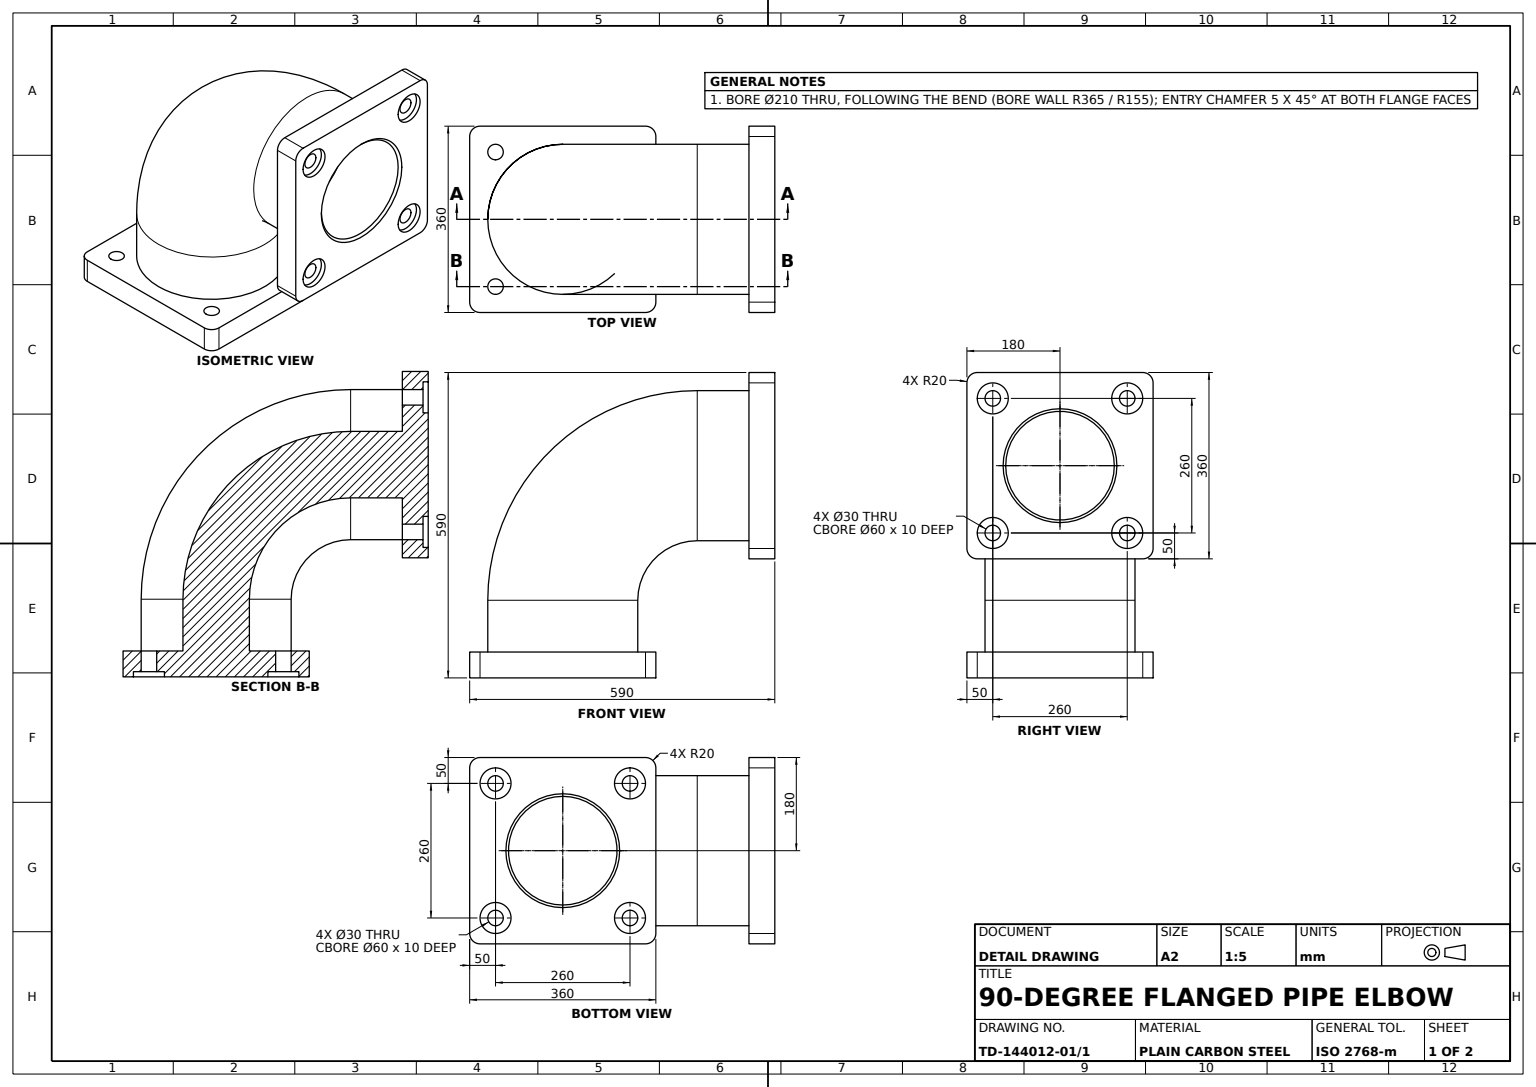
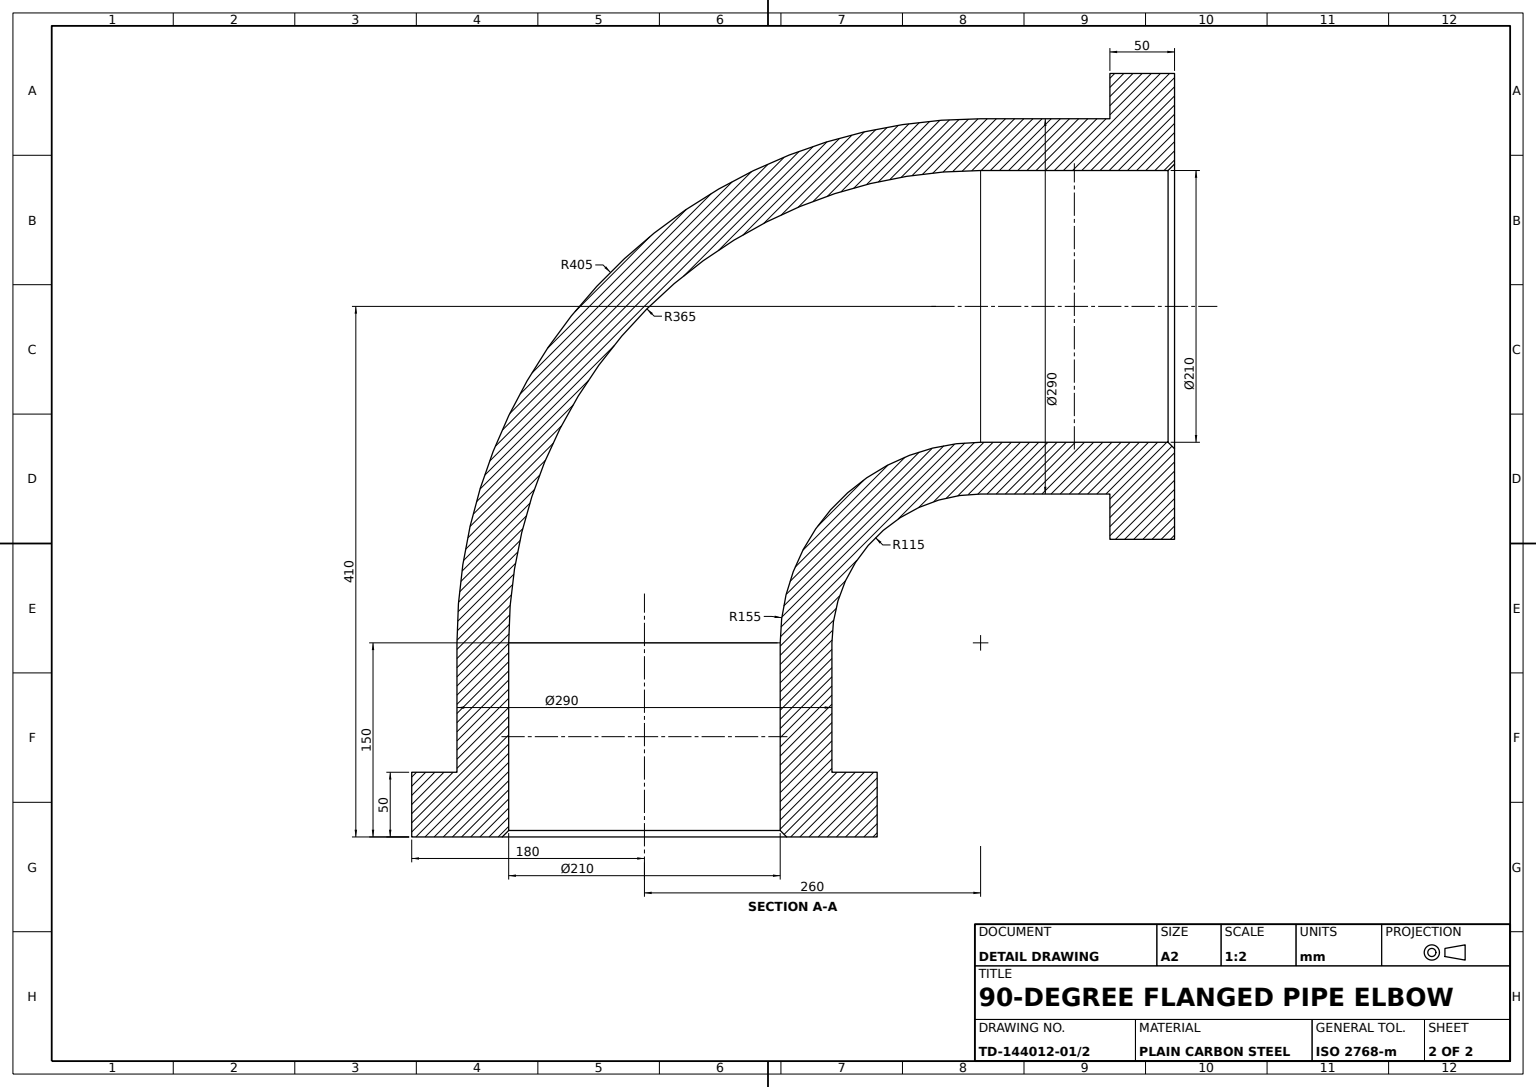
solid
v1 (-130,50,115)
v2 (-130,10,115)
e1 v1 v2 LINE
v3 (-130,50,145)
e2 v3 v1 CIRCLE(AX(P(-130,50,130),D(0,-1,0),D(0,0,-1)),15)
v4 (-130,10,145)
e3 v3 v4 LINE
e4 v2 v4 CIRCLE(AX(P(-130,10,130),D(0,1,0),D(0,0,-1)),15)
face CYL(AX(P(-130,50,130),D(0,-1,0),D(0,0,-1)),15) rev [-e1 -e2 e3 -e4]
v5 (-130,10,100)
v6 (-130,10,160)
e5 v5 v6 CIRCLE(AX(P(-130,10,130),D(0,-1,0),D(0,0,-1)),30)
e6 v6 v5 CIRCLE(AX(P(-130,10,130),D(0,-1,0),D(0,0,-1)),30)
e7 v4 v2 CIRCLE(AX(P(-130,10,130),D(0,1,0),D(0,0,-1)),15)
face PLANE(AX(P(-130,10,130),D(0,-1,0),D(0,0,-1))) [e5 e6] [e7 e4]
v7 (360,540,115)
v8 (400,540,115)
e8 v7 v8 LINE
v9 (400,540,145)
e9 v9 v8 CIRCLE(AX(P(400,540,130),D(-1,0,0),D(0,0,-1)),15)
v10 (360,540,145)
e10 v10 v9 LINE
e11 v7 v10 CIRCLE(AX(P(360,540,130),D(1,0,0),D(0,0,-1)),15)
face CYL(AX(P(360,540,130),D(1,0,0),D(0,0,-1)),15) rev [e8 -e9 -e10 -e11]
v11 (0,0,-110)
v12 (0,0,110)
e12 v11 v12 CIRCLE(AX(P(0,0,0),D(0,1,0),D(0,0,1)),110)
v13 (0,5,-105)
e13 v13 v11 LINE
v14 (0,5,105)
e14 v14 v13 CIRCLE(AX(P(0,5,0),D(0,-1,0),D(0,0,1)),105)
e15 v14 v12 LINE
face CONE(AX(P(0,5,0),D(0,-1,0),D(0,0,-1)),105,0.785398163) rev [-e12 -e13 -e14 e15]
v15 (410,540,160)
v16 (410,540,100)
e16 v15 v16 CIRCLE(AX(P(410,540,130),D(1,0,0),D(0,0,-1)),30)
v17 (400,540,100)
e17 v17 v16 LINE
v18 (400,540,160)
e18 v18 v17 CIRCLE(AX(P(400,540,130),D(1,0,0),D(0,0,-1)),30)
e19 v18 v15 LINE
face CYL(AX(P(400,540,130),D(1,0,0),D(0,0,-1)),30) rev [e16 -e17 -e18 e19]
v19 (0,150,-105)
v20 (105,150,0)
e20 v19 v20 CIRCLE(AX(P(0,150,0),D(0,-1,0),D(0,0,-1)),105)
e21 v13 v19 LINE
e22 v13 v14 CIRCLE(AX(P(0,5,0),D(0,-1,0),D(0,0,1)),105)
v21 (0,150,105)
e23 v14 v21 LINE
e24 v20 v21 CIRCLE(AX(P(0,150,0),D(0,-1,0),D(0,0,-1)),105)
face CYL(AX(P(0,0,0),D(0,1,0),D(0,0,1)),105) rev [-e20 -e21 e22 e23 -e24]
e25 v1 v3 CIRCLE(AX(P(-130,50,130),D(0,-1,0),D(0,0,-1)),15)
face CYL(AX(P(-130,50,130),D(0,-1,0),D(0,0,-1)),15) rev [-e25 e1 -e7 -e3]
v22 (360,280,-115)
v23 (360,280,-145)
e26 v22 v23 CIRCLE(AX(P(360,280,-130),D(1,0,0),D(0,0,1)),15)
v24 (400,280,-115)
e27 v22 v24 LINE
v25 (400,280,-145)
e28 v25 v24 CIRCLE(AX(P(400,280,-130),D(-1,0,0),D(0,0,-1)),15)
e29 v23 v25 LINE
face CYL(AX(P(360,280,-130),D(1,0,0),D(0,0,-1)),15) rev [-e26 e27 -e28 -e29]
v26 (-130,50,-145)
v27 (-130,10,-145)
e30 v26 v27 LINE
v28 (-130,10,-115)
e31 v28 v27 CIRCLE(AX(P(-130,10,-130),D(0,1,0),D(0,0,-1)),15)
v29 (-130,50,-115)
e32 v29 v28 LINE
e33 v26 v29 CIRCLE(AX(P(-130,50,-130),D(0,-1,0),D(0,0,-1)),15)
face CYL(AX(P(-130,50,-130),D(0,-1,0),D(0,0,-1)),15) rev [e30 -e31 -e32 -e33]
v30 (-105,150,0)
e34 v30 v19 CIRCLE(AX(P(0,150,0),D(0,-1,0),D(0,0,-1)),105)
v31 (260,305,0)
e35 v20 v31 CIRCLE(AX(P(260,150,0),D(0,0,-1),D(-1,0,0)),155)
v32 (260,410,-105)
e36 v32 v31 CIRCLE(AX(P(260,410,0),D(-1,0,0),D(0,0,-1)),105)
v33 (260,515,0)
e37 v33 v32 CIRCLE(AX(P(260,410,0),D(-1,0,0),D(0,0,-1)),105)
e38 v30 v33 CIRCLE(AX(P(260,150,0),D(0,0,-1),D(-1,0,0)),365)
face TORUS(AX(P(260,150,0),D(0,0,-1),D(-1,0,0)),260,105) rev [e34 e20 e35 -e36 -e37 -e38]
v34 (400,540,-145)
v35 (400,540,-115)
e39 v34 v35 CIRCLE(AX(P(400,540,-130),D(-1,0,0),D(0,0,-1)),15)
e40 v35 v34 CIRCLE(AX(P(400,540,-130),D(-1,0,0),D(0,0,-1)),15)
v36 (400,540,-100)
v37 (400,540,-160)
e41 v36 v37 CIRCLE(AX(P(400,540,-130),D(1,0,0),D(0,0,-1)),30)
e42 v37 v36 CIRCLE(AX(P(400,540,-130),D(1,0,0),D(0,0,-1)),30)
face PLANE(AX(P(400,540,-130),D(1,0,0),D(0,0,-1))) [e39 e40] [e41 e42]
v38 (360,590,-160)
v39 (360,590,160)
e43 v38 v39 LINE
v40 (410,590,160)
e44 v39 v40 LINE
v41 (410,590,-160)
e45 v41 v40 LINE
e46 v38 v41 LINE
face PLANE(AX(P(360,590,160),D(0,1,0),D(0,0,1))) [e43 e44 -e45 -e46]
v42 (360,570,-180)
v43 (410,570,-180)
e47 v42 v43 LINE
v44 (410,250,-180)
e48 v44 v43 LINE
v45 (360,250,-180)
e49 v45 v44 LINE
e50 v45 v42 LINE
face PLANE(AX(P(360,250,-180),D(0,0,-1),D(-1,0,0))) [e47 -e48 -e49 e50]
v46 (-130,0,100)
v47 (-130,0,160)
e51 v46 v47 CIRCLE(AX(P(-130,0,130),D(0,-1,0),D(0,0,-1)),30)
e52 v6 v47 LINE
e53 v5 v46 LINE
face CYL(AX(P(-130,10,130),D(0,-1,0),D(0,0,-1)),30) rev [e51 -e52 -e5 e53]
e54 v21 v30 CIRCLE(AX(P(0,150,0),D(0,-1,0),D(0,0,-1)),105)
v48 (260,410,105)
e55 v48 v33 CIRCLE(AX(P(260,410,0),D(-1,0,0),D(0,0,-1)),105)
e56 v31 v48 CIRCLE(AX(P(260,410,0),D(-1,0,0),D(0,0,-1)),105)
face TORUS(AX(P(260,150,0),D(0,0,-1),D(-1,0,0)),260,105) rev [-e35 e24 e54 e38 -e55 -e56]
v49 (-130,10,-160)
v50 (-130,0,-160)
e57 v49 v50 LINE
v51 (-130,10,-100)
e58 v51 v49 CIRCLE(AX(P(-130,10,-130),D(0,-1,0),D(0,0,-1)),30)
v52 (-130,0,-100)
e59 v51 v52 LINE
e60 v52 v50 CIRCLE(AX(P(-130,0,-130),D(0,-1,0),D(0,0,-1)),30)
face CYL(AX(P(-130,10,-130),D(0,-1,0),D(0,0,-1)),30) rev [-e57 -e58 e59 e60]
v53 (360,280,145)
v54 (400,280,145)
e61 v53 v54 LINE
v55 (400,280,115)
e62 v55 v54 CIRCLE(AX(P(400,280,130),D(-1,0,0),D(0,0,-1)),15)
v56 (360,280,115)
e63 v56 v55 LINE
e64 v53 v56 CIRCLE(AX(P(360,280,130),D(1,0,0),D(0,0,-1)),15)
face CYL(AX(P(360,280,130),D(1,0,0),D(0,0,-1)),15) rev [e61 -e62 -e63 -e64]
v57 (130,0,100)
v58 (130,0,160)
e65 v57 v58 CIRCLE(AX(P(130,0,130),D(0,-1,0),D(0,0,-1)),30)
e66 v58 v57 CIRCLE(AX(P(130,0,130),D(0,-1,0),D(0,0,-1)),30)
v59 (160,0,180)
v60 (-160,0,180)
e67 v59 v60 LINE
v61 (-180,0,160)
e68 v60 v61 CIRCLE(AX(P(-160,0,160),D(0,-1,0),D(0,0,1)),20)
v62 (-180,0,-160)
e69 v61 v62 LINE
v63 (-160,0,-180)
e70 v62 v63 CIRCLE(AX(P(-160,0,-160),D(0,-1,0),D(0,0,1)),20)
v64 (160,0,-180)
e71 v63 v64 LINE
v65 (180,0,-160)
e72 v64 v65 CIRCLE(AX(P(160,0,-160),D(0,-1,0),D(0,0,-1)),20)
v66 (180,0,160)
e73 v65 v66 LINE
e74 v66 v59 CIRCLE(AX(P(160,0,160),D(0,-1,0),D(0,0,1)),20)
e75 v47 v46 CIRCLE(AX(P(-130,0,130),D(0,-1,0),D(0,0,-1)),30)
e76 v50 v52 CIRCLE(AX(P(-130,0,-130),D(0,-1,0),D(0,0,-1)),30)
v67 (130,0,-160)
v68 (130,0,-100)
e77 v67 v68 CIRCLE(AX(P(130,0,-130),D(0,-1,0),D(0,0,-1)),30)
e78 v68 v67 CIRCLE(AX(P(130,0,-130),D(0,-1,0),D(0,0,-1)),30)
e79 v12 v11 CIRCLE(AX(P(0,0,0),D(0,1,0),D(0,0,1)),110)
face PLANE(AX(P(0,0,0),D(0,1,0),D(0,0,-1))) rev [-e65 -e66] [e67 e68 e69 e70 e71 e72 e73 e74] [-e51 -e75] [-e60 -e76] [-e77 -e78] [e79 e12]
v69 (0,50,145)
v70 (0,50,-145)
e80 v69 v70 CIRCLE(AX(P(0,50,0),D(0,-1,0),D(0,0,1)),145)
e81 v70 v69 CIRCLE(AX(P(0,50,0),D(0,-1,0),D(0,0,1)),145)
e82 v29 v26 CIRCLE(AX(P(-130,50,-130),D(0,-1,0),D(0,0,-1)),15)
v71 (180,50,160)
v72 (160,50,180)
e83 v71 v72 CIRCLE(AX(P(160,50,160),D(0,-1,0),D(0,0,1)),20)
v73 (180,50,-160)
e84 v73 v71 LINE
v74 (160,50,-180)
e85 v74 v73 CIRCLE(AX(P(160,50,-160),D(0,-1,0),D(0,0,-1)),20)
v75 (-160,50,-180)
e86 v75 v74 LINE
v76 (-180,50,-160)
e87 v76 v75 CIRCLE(AX(P(-160,50,-160),D(0,-1,0),D(0,0,1)),20)
v77 (-180,50,160)
e88 v77 v76 LINE
v78 (-160,50,180)
e89 v78 v77 CIRCLE(AX(P(-160,50,160),D(0,-1,0),D(0,0,1)),20)
e90 v72 v78 LINE
v79 (130,50,-115)
v80 (130,50,-145)
e91 v79 v80 CIRCLE(AX(P(130,50,-130),D(0,-1,0),D(0,0,1)),15)
e92 v80 v79 CIRCLE(AX(P(130,50,-130),D(0,-1,0),D(0,0,1)),15)
v81 (130,50,115)
v82 (130,50,145)
e93 v81 v82 CIRCLE(AX(P(130,50,130),D(0,-1,0),D(0,0,1)),15)
e94 v82 v81 CIRCLE(AX(P(130,50,130),D(0,-1,0),D(0,0,1)),15)
face PLANE(AX(P(-160,50,-160),D(0,1,0),D(0,0,1))) [e80 e81] [e82 e33] [e25 e2] [-e83 -e84 -e85 -e86 -e87 -e88 -e89 -e90] [e91 e92] [e93 e94]
e95 v73 v65 LINE
e96 v74 v64 LINE
face CYL(AX(P(160,50,-160),D(0,-1,0),D(0,0,-1)),20) [e95 -e72 -e96 e85]
face CYL(AX(P(0,0,0),D(0,1,0),D(0,0,1)),105) rev [e14 e21 -e34 -e54 -e23]
v83 (400,280,-160)
v84 (410,280,-160)
e97 v83 v84 LINE
v85 (400,280,-100)
e98 v85 v83 CIRCLE(AX(P(400,280,-130),D(1,0,0),D(0,0,-1)),30)
v86 (410,280,-100)
e99 v85 v86 LINE
e100 v86 v84 CIRCLE(AX(P(410,280,-130),D(1,0,0),D(0,0,-1)),30)
face CYL(AX(P(400,280,-130),D(1,0,0),D(0,0,-1)),30) rev [-e97 -e98 e99 e100]
e101 v17 v18 CIRCLE(AX(P(400,540,130),D(1,0,0),D(0,0,-1)),30)
e102 v8 v9 CIRCLE(AX(P(400,540,130),D(-1,0,0),D(0,0,-1)),15)
face PLANE(AX(P(400,540,130),D(1,0,0),D(0,0,-1))) [e101 e18] [e102 e9]
v87 (405,410,105)
v88 (410,410,110)
e103 v87 v88 LINE
v89 (410,410,-110)
e104 v89 v88 CIRCLE(AX(P(410,410,0),D(-1,0,0),D(0,0,-1)),110)
v90 (405,410,-105)
e105 v90 v89 LINE
e106 v87 v90 CIRCLE(AX(P(405,410,0),D(1,0,0),D(0,0,-1)),105)
face CONE(AX(P(410,410,0),D(1,0,0),D(0,0,-1)),110,0.785398163) rev [e103 -e104 -e105 -e106]
e107 v10 v7 CIRCLE(AX(P(360,540,130),D(1,0,0),D(0,0,-1)),15)
face CYL(AX(P(360,540,130),D(1,0,0),D(0,0,-1)),15) rev [-e107 e10 -e102 -e8]
v91 (410,230,160)
v92 (410,230,-160)
e108 v91 v92 LINE
v93 (360,230,160)
e109 v93 v91 LINE
v94 (360,230,-160)
e110 v93 v94 LINE
e111 v94 v92 LINE
face PLANE(AX(P(360,230,160),D(0,-1,0),D(0,0,-1))) [-e108 -e109 e110 e111]
e112 v84 v86 CIRCLE(AX(P(410,280,-130),D(1,0,0),D(0,0,-1)),30)
e113 v83 v85 CIRCLE(AX(P(400,280,-130),D(1,0,0),D(0,0,-1)),30)
face CYL(AX(P(400,280,-130),D(1,0,0),D(0,0,-1)),30) rev [e97 e112 -e99 -e113]
e114 v24 v25 CIRCLE(AX(P(400,280,-130),D(-1,0,0),D(0,0,-1)),15)
face PLANE(AX(P(400,280,-130),D(1,0,0),D(0,0,-1))) [e98 e113] [e114 e28]
e115 v54 v55 CIRCLE(AX(P(400,280,130),D(-1,0,0),D(0,0,-1)),15)
e116 v56 v53 CIRCLE(AX(P(360,280,130),D(1,0,0),D(0,0,-1)),15)
face CYL(AX(P(360,280,130),D(1,0,0),D(0,0,-1)),15) rev [-e115 -e61 -e116 e63]
v95 (360,540,-115)
e117 v95 v35 LINE
v96 (360,540,-145)
e118 v96 v34 LINE
e119 v95 v96 CIRCLE(AX(P(360,540,-130),D(1,0,0),D(0,0,1)),15)
face CYL(AX(P(360,540,-130),D(1,0,0),D(0,0,-1)),15) rev [e117 -e39 -e118 -e119]
e120 v48 v87 LINE
e121 v32 v90 LINE
face CYL(AX(P(260,410,0),D(1,0,0),D(0,0,-1)),105) rev [e36 e56 e120 e106 -e121]
v97 (0,150,-145)
v98 (-145,150,0)
e122 v97 v98 CIRCLE(AX(P(0,150,0),D(0,1,0),D(0,0,-1)),145)
e123 v70 v97 LINE
v99 (0,150,145)
e124 v69 v99 LINE
e125 v98 v99 CIRCLE(AX(P(0,150,0),D(0,1,0),D(0,0,-1)),145)
face CYL(AX(P(0,0,0),D(0,1,0),D(0,0,1)),145) [-e122 -e123 -e80 e124 -e125]
v100 (130,10,100)
e126 v100 v57 LINE
v101 (130,10,160)
e127 v101 v100 CIRCLE(AX(P(130,10,130),D(0,-1,0),D(0,0,-1)),30)
e128 v101 v58 LINE
face CYL(AX(P(130,10,130),D(0,-1,0),D(0,0,-1)),30) rev [e66 -e126 -e127 e128]
v102 (360,570,180)
e129 v39 v102 CIRCLE(AX(P(360,570,160),D(1,0,0),D(0,0,1)),20)
v103 (410,570,180)
e130 v102 v103 LINE
e131 v40 v103 CIRCLE(AX(P(410,570,160),D(1,0,0),D(0,0,1)),20)
face CYL(AX(P(360,570,160),D(1,0,0),D(0,0,-1)),20) [e129 e130 -e131 -e44]
v104 (130,10,-115)
v105 (130,10,-145)
e132 v104 v105 CIRCLE(AX(P(130,10,-130),D(0,1,0),D(0,0,-1)),15)
e133 v105 v104 CIRCLE(AX(P(130,10,-130),D(0,1,0),D(0,0,-1)),15)
v106 (130,10,-160)
v107 (130,10,-100)
e134 v106 v107 CIRCLE(AX(P(130,10,-130),D(0,-1,0),D(0,0,-1)),30)
e135 v107 v106 CIRCLE(AX(P(130,10,-130),D(0,-1,0),D(0,0,-1)),30)
face PLANE(AX(P(130,10,-130),D(0,-1,0),D(0,0,-1))) [e132 e133] [e134 e135]
e136 v71 v66 LINE
face PLANE(AX(P(180,50,-160),D(1,0,0),D(0,0,-1))) [-e95 e84 e136 -e73]
e137 v106 v67 LINE
e138 v107 v68 LINE
face CYL(AX(P(130,10,-130),D(0,-1,0),D(0,0,-1)),30) rev [-e134 e137 e77 -e138]
v108 (130,10,115)
e139 v81 v108 LINE
v109 (130,10,145)
e140 v109 v108 CIRCLE(AX(P(130,10,130),D(0,1,0),D(0,0,-1)),15)
e141 v82 v109 LINE
face CYL(AX(P(130,50,130),D(0,-1,0),D(0,0,-1)),15) rev [-e93 e139 -e140 -e141]
e142 v16 v15 CIRCLE(AX(P(410,540,130),D(1,0,0),D(0,0,-1)),30)
face CYL(AX(P(400,540,130),D(1,0,0),D(0,0,-1)),30) rev [e17 e142 -e19 -e101]
e143 v90 v87 CIRCLE(AX(P(405,410,0),D(1,0,0),D(0,0,-1)),105)
e144 v88 v89 CIRCLE(AX(P(410,410,0),D(-1,0,0),D(0,0,-1)),110)
face CONE(AX(P(410,410,0),D(1,0,0),D(0,0,-1)),110,0.785398163) rev [-e143 e105 -e144 -e103]
e145 v77 v61 LINE
e146 v78 v60 LINE
face CYL(AX(P(-160,50,160),D(0,-1,0),D(0,0,-1)),20) [e89 e145 -e68 -e146]
face CYL(AX(P(130,10,-130),D(0,-1,0),D(0,0,-1)),30) rev [-e137 -e135 e138 e78]
v110 (260,410,145)
v111 (360,410,145)
e147 v110 v111 LINE
v112 (360,410,-145)
e148 v112 v111 CIRCLE(AX(P(360,410,0),D(1,0,0),D(0,0,1)),145)
v113 (260,410,-145)
e149 v113 v112 LINE
v114 (260,555,0)
e150 v113 v114 CIRCLE(AX(P(260,410,0),D(1,0,0),D(0,0,-1)),145)
e151 v114 v110 CIRCLE(AX(P(260,410,0),D(1,0,0),D(0,0,-1)),145)
face CYL(AX(P(260,410,0),D(1,0,0),D(0,0,-1)),145) [e147 -e148 -e149 e150 e151]
e152 v72 v59 LINE
face PLANE(AX(P(-160,50,180),D(0,0,1),D(1,0,0))) [e146 -e67 -e152 e90]
e153 v23 v22 CIRCLE(AX(P(360,280,-130),D(1,0,0),D(0,0,1)),15)
face CYL(AX(P(360,280,-130),D(1,0,0),D(0,0,-1)),15) rev [-e27 -e153 e29 -e114]
v115 (145,150,0)
v116 (260,265,0)
e154 v115 v116 CIRCLE(AX(P(260,150,0),D(0,0,-1),D(-1,0,0)),115)
e155 v110 v116 CIRCLE(AX(P(260,410,0),D(1,0,0),D(0,0,-1)),145)
e156 v98 v114 CIRCLE(AX(P(260,150,0),D(0,0,-1),D(-1,0,0)),405)
e157 v99 v115 CIRCLE(AX(P(0,150,0),D(0,1,0),D(0,0,-1)),145)
face TORUS(AX(P(260,150,0),D(0,0,-1),D(-1,0,0)),260,145) [e154 -e155 -e151 -e156 e125 e157]
face CYL(AX(P(260,410,0),D(1,0,0),D(0,0,-1)),105) rev [e55 e37 e121 e143 -e120]
e158 v100 v101 CIRCLE(AX(P(130,10,130),D(0,-1,0),D(0,0,-1)),30)
face CYL(AX(P(130,10,130),D(0,-1,0),D(0,0,-1)),30) rev [e126 e65 -e128 -e158]
e159 v116 v113 CIRCLE(AX(P(260,410,0),D(1,0,0),D(0,0,-1)),145)
e160 v111 v112 CIRCLE(AX(P(360,410,0),D(1,0,0),D(0,0,1)),145)
face CYL(AX(P(260,410,0),D(1,0,0),D(0,0,-1)),145) [e155 e159 e149 -e160 -e147]
e161 v108 v109 CIRCLE(AX(P(130,10,130),D(0,1,0),D(0,0,-1)),15)
face PLANE(AX(P(130,10,130),D(0,-1,0),D(0,0,-1))) [e158 e127] [e140 e161]
face CYL(AX(P(-130,10,130),D(0,-1,0),D(0,0,-1)),30) rev [e75 -e53 -e6 e52]
v117 (410,540,-100)
v118 (410,540,-160)
e162 v117 v118 CIRCLE(AX(P(410,540,-130),D(1,0,0),D(0,0,-1)),30)
e163 v37 v118 LINE
e164 v36 v117 LINE
face CYL(AX(P(400,540,-130),D(1,0,0),D(0,0,-1)),30) rev [e162 -e163 -e41 e164]
e165 v115 v97 CIRCLE(AX(P(0,150,0),D(0,1,0),D(0,0,-1)),145)
face CYL(AX(P(0,0,0),D(0,1,0),D(0,0,1)),145) [-e165 -e157 -e124 -e81 e123]
face CYL(AX(P(130,50,130),D(0,-1,0),D(0,0,-1)),15) rev [-e139 -e94 e141 -e161]
v119 (400,280,100)
v120 (400,280,160)
e166 v119 v120 CIRCLE(AX(P(400,280,130),D(1,0,0),D(0,0,-1)),30)
e167 v120 v119 CIRCLE(AX(P(400,280,130),D(1,0,0),D(0,0,-1)),30)
face PLANE(AX(P(400,280,130),D(1,0,0),D(0,0,-1))) [e62 e115] [e166 e167]
e168 v76 v62 LINE
face PLANE(AX(P(-180,50,-160),D(-1,0,0),D(0,0,1))) [e88 e168 -e69 -e145]
e169 v75 v63 LINE
face PLANE(AX(P(-160,50,-180),D(0,0,-1),D(-1,0,0))) [-e169 e86 e96 -e71]
v121 (410,280,160)
v122 (410,280,100)
e170 v121 v122 CIRCLE(AX(P(410,280,130),D(1,0,0),D(0,0,-1)),30)
e171 v119 v122 LINE
e172 v120 v121 LINE
face CYL(AX(P(400,280,130),D(1,0,0),D(0,0,-1)),30) rev [e170 -e171 -e167 e172]
face CONE(AX(P(0,5,0),D(0,-1,0),D(0,0,-1)),105,0.785398163) rev [-e22 e13 -e79 -e15]
v123 (360,250,180)
e173 v123 v93 CIRCLE(AX(P(360,250,160),D(1,0,0),D(0,0,1)),20)
v124 (410,250,180)
e174 v124 v91 CIRCLE(AX(P(410,250,160),D(1,0,0),D(0,0,1)),20)
e175 v123 v124 LINE
face CYL(AX(P(360,250,160),D(1,0,0),D(0,0,-1)),20) [e173 e109 -e174 -e175]
e176 v79 v104 LINE
e177 v80 v105 LINE
face CYL(AX(P(130,50,-130),D(0,-1,0),D(0,0,-1)),15) rev [-e176 -e92 e177 -e132]
e178 v102 v123 LINE
e179 v103 v124 LINE
face PLANE(AX(P(360,250,180),D(0,0,1),D(1,0,0))) [e178 e175 -e179 -e130]
e180 v122 v121 CIRCLE(AX(P(410,280,130),D(1,0,0),D(0,0,-1)),30)
face CYL(AX(P(400,280,130),D(1,0,0),D(0,0,-1)),30) rev [e171 e180 -e172 -e166]
e181 v27 v28 CIRCLE(AX(P(-130,10,-130),D(0,1,0),D(0,0,-1)),15)
face CYL(AX(P(-130,50,-130),D(0,-1,0),D(0,0,-1)),15) rev [-e30 -e82 e32 -e181]
e182 v96 v95 CIRCLE(AX(P(360,540,-130),D(1,0,0),D(0,0,1)),15)
face CYL(AX(P(360,540,-130),D(1,0,0),D(0,0,-1)),15) rev [-e117 -e182 e118 -e40]
e183 v92 v44 CIRCLE(AX(P(410,250,-160),D(1,0,0),D(0,0,-1)),20)
e184 v43 v41 CIRCLE(AX(P(410,570,-160),D(1,0,0),D(0,0,1)),20)
e185 v118 v117 CIRCLE(AX(P(410,540,-130),D(1,0,0),D(0,0,-1)),30)
face PLANE(AX(P(410,410,0),D(1,0,0),D(0,0,-1))) [e144 e104] [-e180 -e170] [-e112 -e100] [e131 e179 e174 e108 e183 e48 e184 e45] [-e185 -e162] [-e16 -e142]
face CYL(AX(P(-160,50,-160),D(0,-1,0),D(0,0,-1)),20) [e169 -e70 -e168 e87]
e186 v49 v51 CIRCLE(AX(P(-130,10,-130),D(0,-1,0),D(0,0,-1)),30)
face CYL(AX(P(-130,10,-130),D(0,-1,0),D(0,0,-1)),30) rev [e57 e76 -e59 -e186]
face PLANE(AX(P(-130,10,-130),D(0,-1,0),D(0,0,-1))) [e186 e58] [e31 e181]
face TORUS(AX(P(260,150,0),D(0,0,-1),D(-1,0,0)),260,145) [-e154 e165 e122 e156 -e150 -e159]
e187 v42 v38 CIRCLE(AX(P(360,570,-160),D(1,0,0),D(0,0,1)),20)
face CYL(AX(P(360,570,-160),D(1,0,0),D(0,0,-1)),20) [-e184 -e47 e187 e46]
e188 v94 v45 CIRCLE(AX(P(360,250,-160),D(1,0,0),D(0,0,-1)),20)
face CYL(AX(P(360,250,-160),D(1,0,0),D(0,0,-1)),20) [-e111 e188 e49 -e183]
face CYL(AX(P(400,540,-130),D(1,0,0),D(0,0,-1)),30) rev [e185 -e164 -e42 e163]
face CYL(AX(P(160,50,160),D(0,-1,0),D(0,0,-1)),20) [e152 -e74 -e136 e83]
face CYL(AX(P(130,50,-130),D(0,-1,0),D(0,0,-1)),15) rev [e176 -e133 -e177 -e91]
face PLANE(AX(P(360,570,160),D(-1,0,0),D(0,0,1))) [e148 e160] [e11 e107] [e116 e64] [e119 e182] [e26 e153] [-e187 -e50 -e188 -e110 -e173 -e178 -e129 -e43]
